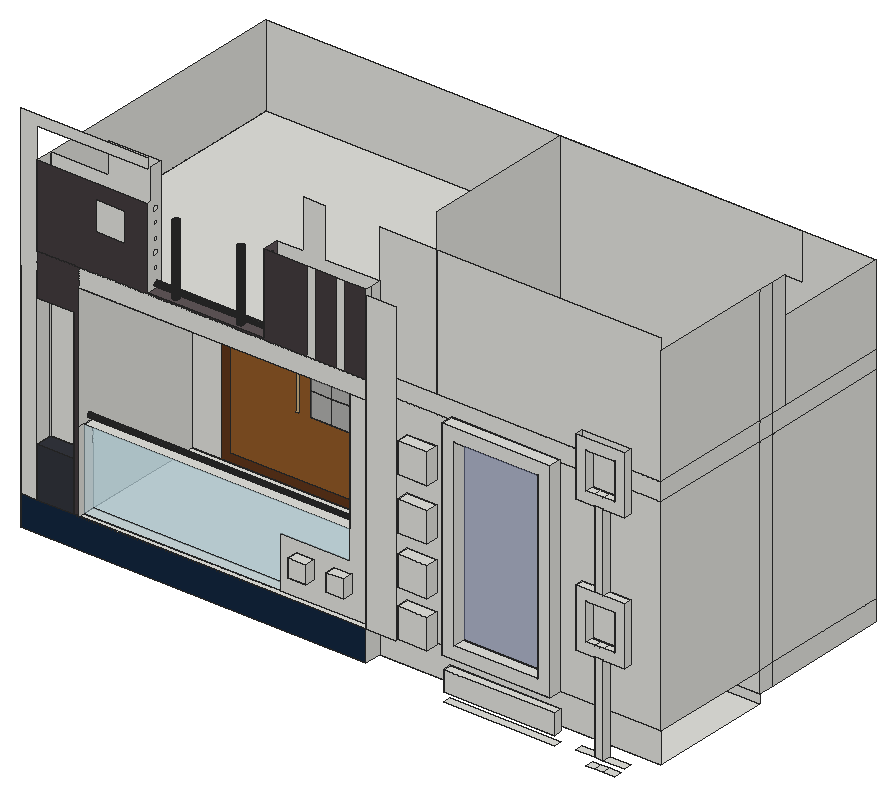
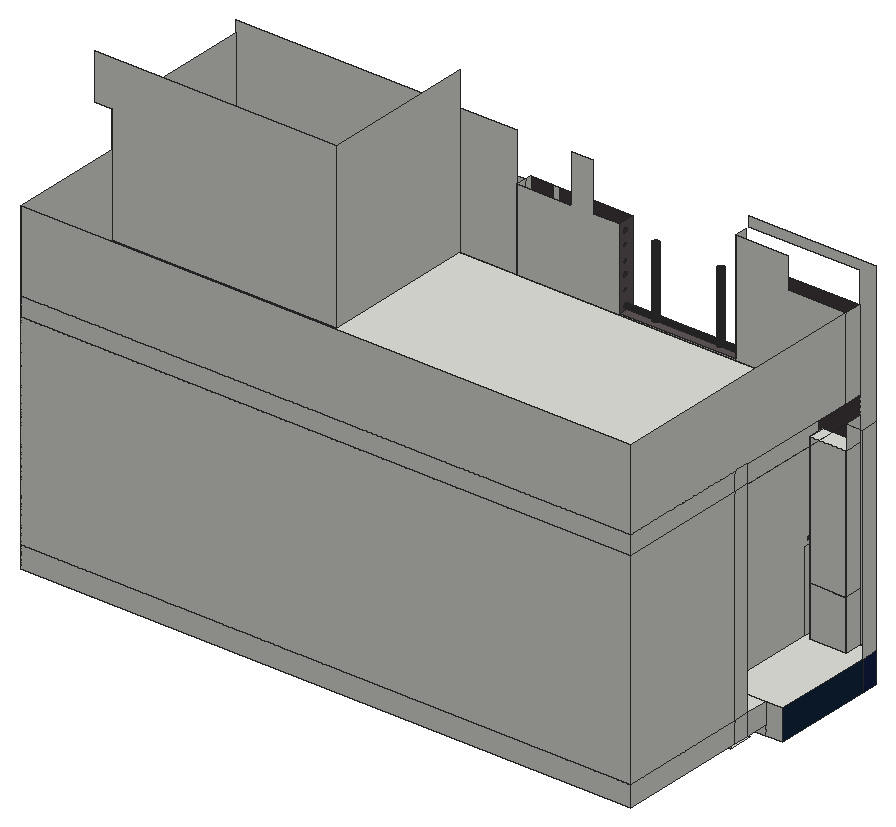
# SketchUp Ruby script. Lengths in inches.
U = 1.inch
M = Sketchup.active_model
def pt(a) = Geom::Point3d.new(a.map { |v| v * U })
def face(e, loops, mat)
  f = e.add_face(loops[0].map { |a| pt(a) })
  loops[1..].each { |l| e.add_face(l.map { |a| pt(a) }).erase! }
  f.material = f.back_material = mat if mat
  f
end
# faces: each face lists its corners as indices into pts; further lists are holes
def faces(e, pts, list, mat = nil) = list.each { |f| face(e, (f[0].is_a?(Array) ? f : [f]).map { |l| l.map { |i| pts[i] } }, mat) }
# xy, xz, yz: faces in a plane at the given z, y or x. An outline is a flat list of corners, or four numbers for a rectangle; further outlines are holes
def ring(l) = l.size == 4 ? [[l[0], l[1]], [l[2], l[1]], [l[2], l[3]], [l[0], l[3]]] : l.each_slice(2).to_a
def flat(e, list, mat, &to3) = list.each { |f| face(e, (f[0].is_a?(Array) ? f : [f]).map { |l| ring(l).map { |u, v| to3.(u, v) } }, mat) }
def xy(e, z, list, mat = nil) = flat(e, list, mat) { |x, y| [x, y, z] }
def xz(e, y, list, mat = nil) = flat(e, list, mat) { |x, z| [x, y, z] }
def yz(e, x, list, mat = nil) = flat(e, list, mat) { |y, z| [x, y, z] }
def lines(e, pts, list) = list.each { |a, b| e.add_line(pt(pts[a]), pt(pts[b])) }
# prism: a flat outline (further loops are holes) pulled along v
def prism(e, loops, v, mat = nil)
  f = face(e, loops, mat); d = Geom::Vector3d.new(v.map { |x| x * U })
  f.pushpull(f.normal.samedirection?(d) ? d.length : -d.length)
end
def box(e, o, s, mat = nil) = prism(e, [[o, [o[0] + s[0], o[1], o[2]], [o[0] + s[0], o[1] + s[1], o[2]], [o[0], o[1] + s[1], o[2]]]], [0, 0, s[2]], mat)
def at(x, y, z, deg = 0) = Geom::Transformation.translation(pt([x, y, z])) * Geom::Transformation.rotation(ORIGIN, Z_AXIS, deg.degrees)
def axes(o, x, y, z) = Geom::Transformation.new([*x, 0, *y, 0, *z, 0, *pt(o).to_a, 1])
def part(name) = M.definitions.add(name)
# library, detail: a bought-in or finely detailed component or shape, given as its bounding box
def library(name, o, s) = part(name).tap { |d| box(d.entities, o, s) }
def detail(e, o, s) = box(e.add_group.entities, o, s)
def put(e, d, t, mat = nil) = e.add_instance(d, t).tap { |i| i.material = mat if mat }
def group(e, t, mat = nil) = e.add_group.tap { |g| g.transformation = t; g.material = mat if mat }.entities
root = M.entities
M.materials.add("[Asphalt New]").color = [96, 86, 89]
M.materials.add("[Asphalt New]1").color = [67, 60, 62]
M.materials.add("[Carrera Marble]").color = [19, 39, 63]
M.materials.add("[Color M07]").color = [58, 58, 58]
M.materials.add("[Formica Laminate Dark]").color = [50, 53, 60]
M.materials.add("[Granite Dark Gray]").color = [18, 32, 73]
M.materials.add("[Translucent Glass Gray]").color = [128, 128, 128]
M.materials["[Translucent Glass Gray]"].alpha = 0.5
M.materials.add("[Translucent Glass Safety]").color = [213, 245, 255]
M.materials["[Translucent Glass Safety]"].alpha = 0.5
M.materials.add("[Translucent Glass Sky Reflection]").color = [126, 138, 183]
M.materials["[Translucent Glass Sky Reflection]"].alpha = 0.52
M.materials.add("[Wood Cherry Original]").color = [96, 54, 26]
M.materials.add("[Wood Floor Light]").color = [204, 176, 127]
M.materials.add("[Wood Floor Parquet]").color = [145, 89, 39]
box(root,[294.43,147.85,88.67],[58.93,4.5,10.68])
box(root,[271.51,145.85,106.65],[15.82,6.5,15.81])
box(root,[271.51,145.85,131.4],[15.82,6.5,15.81])
box(root,[271.51,145.85,157.4],[15.82,6.5,15.81])
box(root,[271.51,145.85,185.28],[15.82,6.5,15.81])
xy(root,80.14,[[370.09,148.04,374.5,152.35],[374.5,148.04,379.09,152.35],[379.09,148.04,385.11,152.35]])
xy(root,81.17,[[83.43,214.25,224.39,226.93]])
xy(root,83.85,[[294.43,147.85,353.36,152.35]])
xy(root,84.875,[[65.99,152.35,65.99,214.25,241.35,214.25,241.35,226.93,399.27,226.93,399.27,161.35,249.72,161.35,249.72,152.35]])
xy(root,85.66,[[364.57,148.04,374.5,152.35],[374.5,148.04,379.09,152.35],[379.09,148.04,390.63,152.35]])
xy(root,89.9375,[[74.99,214.25,241.35,226.93],[74.99,226.93,399.27,234.75],[74.99,234.75,399.27,304.28]])
xy(root,101,[[65.99,152.35,74.71,152.35,74.71,161.47,94.21,161.47,94.21,152.35,97.3,152.35,97.3,214.25,65.99,214.25],[74.71,152.35,94.21,161.47],[97.3,152.35,249.72,155.29],[97.3,155.29,249.72,161.35],[97.3,161.35,399.27,226.93],
  [74.99,214.25,97.3,226.93],[74.99,226.93,399.27,234.75],[74.99,234.75,399.27,304.28]])
xy(root,107.34,[[295.03,145.79,352.78,152.35]])
xy(root,112.78,[[210.38,149.85,219.82,155.29],[230.45,149.85,239.88,155.29]])
xy(root,113.91,[[301.6,145.79,346.21,152.35]])
xy(root,122.22,[[210.38,149.85,219.82,155.29],[230.45,149.85,239.88,155.29]])
xy(root,127.5,[[74.71,152.35,94.21,161.47]],"[Formica Laminate Dark]")
xy(root,133.35,[[364.57,148.04,374.5,152.35],[374.5,148.04,379.09,152.35],[379.09,148.04,390.63,152.35]])
xy(root,138.86,[[370.09,148.04,374.5,152.35],[374.5,148.04,379.09,152.35],[379.09,148.04,385.11,152.35]])
xy(root,143.5625,[[97.3,155.29,238.69,161.35]])
xy(root,158.64,[[370.09,148.04,374.5,152.35],[374.5,148.04,379.09,152.35],[379.09,148.04,385.11,152.35]])
xy(root,164.16,[[364.57,148.04,374.5,152.35],[374.5,148.04,379.09,152.35],[379.09,148.04,390.63,152.35]])
xy(root,197.27,[[74.71,152.35,94.21,161.47]])
xy(root,205.28,[[364.57,148.04,374.5,152.35],[374.5,148.04,379.09,152.35],[379.09,148.04,390.63,152.35]])
xy(root,209.9375,[[97.3,152.35,97.3,226.93,399.27,226.93,399.27,161.35,238.69,161.35,238.69,152.35],[238.69,152.35,249.72,155.29],[238.69,155.29,249.72,161.35],[74.99,226.93,399.27,234.75],[74.99,234.75,399.27,304.28]])
xy(root,210.8,[[370.09,148.04,374.5,152.35],[374.5,148.04,379.09,152.35],[379.09,148.04,385.11,152.35]])
xy(root,211.08,[[301.6,145.79,346.21,152.35]])
xy(root,217.65,[[295.03,145.79,352.78,152.35]])
xy(root,219.625,[[74.99,152.35,249.72,161.35],[74.99,161.35,280.02,161.35,280.02,243.33,399.27,243.33,399.27,304.28,74.99,304.28],[280.02,161.35,399.27,243.33]])
xy(root,220.1875,[[145.55,154.65,145.15,154.7,144.77,154.86,144.45,155.11,144.2,155.43,144.04,155.81,143.99,156.21,144.04,156.62,144.2,156.99,144.45,157.32,144.77,157.57,145.15,157.72,145.55,157.77,145.96,157.72,146.33,157.57,146.66,157.32,146.9,156.99,147.0625,156.62,147.11,156.21,147.0625,155.81,146.9,155.43,146.66,155.11,146.33,154.86,145.96,154.7],[180.11,154.65,179.71,154.7,179.33,154.86,179.01,155.11,178.76,155.43,178.6,155.81,178.55,156.21,178.6,156.62,178.76,156.99,179.01,157.32,179.33,157.57,179.71,157.72,180.11,157.77,180.52,157.72,180.9,157.57,181.22,157.32,181.47,156.99,181.625,156.62,181.68,156.21,181.625,155.81,181.47,155.43,181.22,155.11,180.9,154.86,180.52,154.7]])
xy(root,220.1875,[[[133.58,152.35,195.29,161.35],[145.55,154.65,145.15,154.7,144.77,154.86,144.45,155.11,144.2,155.43,144.04,155.81,143.99,156.21,144.04,156.62,144.2,156.99,144.45,157.32,144.77,157.57,145.15,157.72,145.55,157.77,145.96,157.72,146.33,157.57,146.66,157.32,146.9,156.99,147.0625,156.62,147.11,156.21,147.0625,155.81,146.9,155.43,146.66,155.11,146.33,154.86,145.96,154.7],[180.11,154.65,179.71,154.7,179.33,154.86,179.01,155.11,178.76,155.43,178.6,155.81,178.55,156.21,178.6,156.62,178.76,156.99,179.01,157.32,179.33,157.57,179.71,157.72,180.11,157.77,180.52,157.72,180.9,157.57,181.22,157.32,181.47,156.99,181.625,156.62,181.68,156.21,181.625,155.81,181.47,155.43,181.22,155.11,180.9,154.86,180.52,154.7]]],"[Asphalt New]")
xz(root,145.79,[[[295.03,107.34,352.78,217.65],[301.6,113.91,346.21,211.08]]])
xz(root,148.04,[[374.5,85.66,379.09,133.35],[[364.57,133.35,390.63,164.16],[370.09,138.86,385.11,158.64]],[374.5,164.16,379.09,205.28],[[364.57,205.28,390.63,236.1],[370.09,210.8,385.11,230.58]]])
xz(root,149.85,[[210.38,112.78,219.82,122.22],[230.45,112.78,239.88,122.22]])
xz(root,152.35,[[374.5,85.66,379.09,133.35],[65.99,101,74.71,101,74.71,209.9375,74.99,219.625,74.99,279.1,133.58,279.1,133.58,284.4375,65.99,284.4375],[249.72,101,265.65,260.08],[[295.03,107.34,352.78,217.65],[301.6,113.91,346.21,211.08]],[[364.57,133.35,390.63,164.16],[370.09,138.86,385.11,158.64]],
  [370.09,138.86,385.11,158.64],[374.5,164.16,379.09,205.28],[[364.57,205.28,390.63,236.1],[370.09,210.8,385.11,230.58]],[97.3,209.9375,249.72,219.625],[370.09,210.8,385.11,230.58],
  [218.4,219.625,222.46,262.6875],[233.96,219.625,238.02,262.6875]])
xz(root,152.35,[[94.21,101,97.3,101,97.3,219.625,74.99,219.625,74.71,209.9375,74.71,197.27,94.21,197.27],[[74.99,219.625,218.4,219.625,218.4,262.6875,195.29,262.6875,195.29,220.1875,133.58,220.1875,133.58,262.6875,74.99,262.6875],[105.86,239.3,121.54,254.99]],[222.46,219.625,233.96,262.6875],[238.02,219.625,249.72,262.6875]],"[Asphalt New]1")
xz(root,152.35,[[65.99,84.875,249.72,101]],"[Carrera Marble]")
xz(root,152.35,[[74.71,101,94.21,127.5]],"[Formica Laminate Dark]")
xz(root,152.35,[[301.6,113.91,346.21,211.08]],"[Translucent Glass Sky Reflection]")
xz(root,155.29,[[[201.94,101,249.72,101,249.72,209.9375,238.69,209.9375,238.69,128.1875,201.94,128.1875],[210.38,112.78,219.82,122.22],[230.45,112.78,239.88,122.22]],[210.38,112.78,219.82,122.22],[230.45,112.78,239.88,122.22]])
xz(root,155.29,[[97.3,101,201.94,101,201.94,128.1875,238.69,128.1875,238.69,143.5625,97.3,143.5625]],"[Translucent Glass Safety]")
xz(root,161.35,[[249.72,84.875,399.27,101],[249.72,101,399.27,209.9375],[249.72,209.9375,399.27,219.625],[74.99,219.625,74.99,262.6875,106.04,262.6875,106.04,279.1,133.58,279.1,133.58,220.1875,195.29,220.1875,195.29,262.6875,209.34,262.6875,209.34,288.3125,220.78,288.3125,220.78,262.6875,249.72,262.6875,249.72,219.625],[249.72,219.625,280.02,288.3125],
  [280.02,219.625,399.27,288.3125]])
xz(root,161.35,[[97.3,101,97.3,143.5625,238.69,143.5625,238.69,209.9375,249.72,209.9375,249.72,101]],"[Translucent Glass Safety]")
xz(root,161.47,[[74.71,101,94.21,127.5],[74.71,127.5,94.21,197.27]])
xz(root,214.25,[[65.99,84.875,74.99,101],[74.99,84.875,241.35,89.9375]])
xz(root,226.93,[[83.43,81.17,224.39,89.9375],[241.35,84.875,399.27,89.9375],[74.99,89.9375,399.27,101],[74.99,101,97.3,209.9375],[97.3,101,113.07,101,113.07,192.125,188.51,192.125,188.51,101,399.27,101,399.27,209.9375,97.3,209.9375]])
xz(root,226.93,[[160.69,137.52,172.08,150.1],[172.08,137.52,183.47,150.1],[160.69,150.1,172.08,162.67],[172.08,150.1,183.47,162.67],[160.69,162.67,172.08,175.46],
  [172.08,162.67,183.47,175.46],[160.69,175.46,172.08,187.08],[172.08,175.46,183.47,187.08]],"[Translucent Glass Gray]")
xz(root,226.93,[[[113.07,101,188.51,192.125],[118.11,106.04,183.47,187.08]]],"[Wood Cherry Original]")
xz(root,226.93,[[152.7,137.52,155.05,157.98]],"[Wood Floor Light]")
xz(root,226.93,[[[118.11,106.04,183.47,106.04,183.47,137.52,160.69,137.52,160.69,187.08,118.11,187.08],[152.7,137.52,155.05,157.98]]],"[Wood Floor Parquet]")
xz(root,234.75,[[74.99,89.9375,399.27,101],[74.99,101,399.27,209.9375]])
xz(root,243.33,[[280.02,219.625,280.02,306.375,408.27,306.375,408.27,281.9375,399.27,281.9375,399.27,219.625]])
xz(root,304.28,[[74.99,89.9375,399.27,101],[74.99,101,399.27,209.9375],[74.99,209.9375,399.27,219.625],[74.99,219.625,399.27,262.6875]])
yz(root,65.99,[[152.35,101,161.35,209.9375]])
yz(root,65.99,[[161.35,84.875,214.25,101]],"[Carrera Marble]")
yz(root,65.99,[[152.35,84.875,161.35,101]],"[Granite Dark Gray]")
yz(root,74.71,[[152.35,101,161.35,127.5],[161.35,101,161.47,127.5],[152.35,127.5,161.35,197.27],[161.35,127.5,161.47,197.27],[152.35,197.27,161.35,209.9375]])
yz(root,74.99,[[214.25,89.9375,226.93,101],[226.93,89.9375,234.75,101],[234.75,89.9375,304.28,101],[226.93,101,234.75,209.9375],[234.75,101,304.28,209.9375],
  [226.93,209.9375,234.75,219.625],[234.75,209.9375,304.28,219.625],[152.35,219.625,161.35,262.6875],[161.35,219.625,304.28,262.6875]])
yz(root,94.21,[[152.35,101,161.47,127.5],[152.35,127.5,161.47,197.27]])
yz(root,97.3,[[152.35,101,155.29,143.5625],[[161.35,101,226.93,101,226.93,209.9375,152.35,209.9375,152.35,143.5625,161.35,143.5625],[158.43,145.79,158.16,145.83,157.9,145.9375,157.68,146.11,157.51,146.33,157.41,146.58,157.37,146.86,157.41,147.13,157.51,147.39,157.68,147.61,157.9,147.78,158.16,147.88,158.43,147.92,158.71,147.88,158.96,147.78,159.18,147.61,159.35,147.39,159.46,147.13,159.49,146.86,159.46,146.58,159.35,146.33,159.18,146.11,158.96,145.9375,158.71,145.83]],[155.29,101,161.35,143.5625]])
yz(root,133.58,[[[152.35,220.1875,161.35,220.1875,161.35,279.1,154.79,279.1,154.79,262.6875,152.35,262.6875],[157.4,256.53,156.97,256.58,156.5625,256.75,156.21,257.02,155.94,257.37,155.77,257.78,155.72,258.21,155.77,258.65,155.94,259.06,156.21,259.41,156.5625,259.68,156.97,259.84,157.4,259.9,157.84,259.84,158.25,259.68,158.6,259.41,158.87,259.06,159.03,258.65,159.09,258.21,159.03,257.78,158.87,257.37,158.6,257.02,158.25,256.75,157.84,256.58],[157.4,235.59,156.97,235.65,156.5625,235.82,156.21,236.08,155.94,236.43,155.77,236.84,155.72,237.28,155.77,237.71,155.94,238.12,156.21,238.47,156.5625,238.74,156.97,238.91,157.4,238.96,157.84,238.91,158.25,238.74,158.6,238.47,158.87,238.12,159.03,237.71,159.09,237.28,159.03,236.84,158.87,236.43,158.6,236.08,158.25,235.82,157.84,235.65],[157.64,221.32,157.33,221.36,157.04,221.47,156.8,221.66,156.61,221.91,156.49,222.2,156.45,222.5,156.49,222.8125,156.61,223.1,156.8,223.34,157.04,223.53,157.33,223.65,157.64,223.69,157.94,223.65,158.23,223.53,158.48,223.34,158.67,223.1,158.78,222.8125,158.82,222.5,158.78,222.2,158.67,221.91,158.48,221.66,158.23,221.47,157.94,221.36],[157.64,228.69,157.33,228.73,157.04,228.85,156.8,229.04,156.61,229.28,156.49,229.57,156.45,229.88,156.49,230.1875,156.61,230.47,156.8,230.72,157.04,230.91,157.33,231.03,157.64,231.07,157.94,231.03,158.23,230.91,158.48,230.72,158.67,230.47,158.78,230.1875,158.82,229.88,158.78,229.57,158.67,229.28,158.48,229.04,158.23,228.85,157.94,228.73],[157.64,242.44,157.33,242.48,157.04,242.6,156.8,242.79,156.61,243.03,156.49,243.32,156.45,243.63,156.49,243.9375,156.61,244.22,156.8,244.47,157.04,244.66,157.33,244.78,157.64,244.82,157.94,244.78,158.23,244.66,158.48,244.47,158.67,244.22,158.78,243.9375,158.82,243.63,158.78,243.32,158.67,243.03,158.48,242.79,158.23,242.6,157.94,242.48],[157.64,250.38,157.33,250.42,157.04,250.54,156.8,250.73,156.61,250.97,156.49,251.26,156.45,251.57,156.49,251.875,156.61,252.16,156.8,252.41,157.04,252.59,157.33,252.71,157.64,252.75,157.94,252.71,158.23,252.59,158.48,252.41,158.67,252.16,158.78,251.875,158.82,251.57,158.78,251.26,158.67,250.97,158.48,250.73,158.23,250.54,157.94,250.42]]])
yz(root,195.29,[[[152.35,220.1875,161.35,262.6875],[157.4,235.59,157.84,235.65,158.25,235.82,158.6,236.08,158.87,236.43,159.03,236.84,159.09,237.28,159.03,237.71,158.87,238.12,158.6,238.47,158.25,238.74,157.84,238.91,157.4,238.96,156.97,238.91,156.5625,238.74,156.21,238.47,155.94,238.12,155.77,237.71,155.72,237.28,155.77,236.84,155.94,236.43,156.21,236.08,156.5625,235.82,156.97,235.65],[157.4,256.53,157.84,256.58,158.25,256.75,158.6,257.02,158.87,257.37,159.03,257.78,159.09,258.21,159.03,258.65,158.87,259.06,158.6,259.41,158.25,259.68,157.84,259.84,157.4,259.9,156.97,259.84,156.5625,259.68,156.21,259.41,155.94,259.06,155.77,258.65,155.72,258.21,155.77,257.78,155.94,257.37,156.21,257.02,156.5625,256.75,156.97,256.58],[157.64,242.44,157.94,242.48,158.23,242.6,158.48,242.79,158.67,243.03,158.78,243.32,158.82,243.63,158.78,243.9375,158.67,244.22,158.48,244.47,158.23,244.66,157.94,244.78,157.64,244.82,157.33,244.78,157.04,244.66,156.8,244.47,156.61,244.22,156.49,243.9375,156.45,243.63,156.49,243.32,156.61,243.03,156.8,242.79,157.04,242.6,157.33,242.48],[157.64,250.38,157.94,250.42,158.23,250.54,158.48,250.73,158.67,250.97,158.78,251.26,158.82,251.57,158.78,251.875,158.67,252.16,158.48,252.41,158.23,252.59,157.94,252.71,157.64,252.75,157.33,252.71,157.04,252.59,156.8,252.41,156.61,252.16,156.49,251.875,156.45,251.57,156.49,251.26,156.61,250.97,156.8,250.73,157.04,250.54,157.33,250.42],[157.64,228.69,157.94,228.73,158.23,228.85,158.48,229.04,158.67,229.28,158.78,229.57,158.82,229.88,158.78,230.1875,158.67,230.47,158.48,230.72,158.23,230.91,157.94,231.03,157.64,231.07,157.33,231.03,157.04,230.91,156.8,230.72,156.61,230.47,156.49,230.1875,156.45,229.88,156.49,229.57,156.61,229.28,156.8,229.04,157.04,228.85,157.33,228.73],[157.64,221.32,157.94,221.36,158.23,221.47,158.48,221.66,158.67,221.91,158.78,222.2,158.82,222.5,158.78,222.8125,158.67,223.1,158.48,223.34,158.23,223.53,157.94,223.65,157.64,223.69,157.33,223.65,157.04,223.53,156.8,223.34,156.61,223.1,156.49,222.8125,156.45,222.5,156.49,222.2,156.61,221.91,156.8,221.66,157.04,221.47,157.33,221.36]],[157.64,221.32,157.94,221.36,158.23,221.47,158.48,221.66,158.67,221.91,158.78,222.2,158.82,222.5,158.78,222.8125,158.67,223.1,158.48,223.34,158.23,223.53,157.94,223.65,157.64,223.69,157.33,223.65,157.04,223.53,156.8,223.34,156.61,223.1,156.49,222.8125,156.45,222.5,156.49,222.2,156.61,221.91,156.8,221.66,157.04,221.47,157.33,221.36]],"[Asphalt New]")
yz(root,210.38,[[149.85,112.78,155.29,122.22]])
yz(root,219.82,[[149.85,112.78,155.29,122.22]])
yz(root,230.45,[[149.85,112.78,155.29,122.22]])
yz(root,238.69,[[[155.29,143.5625,161.35,209.9375],[158.43,145.79,158.71,145.83,158.96,145.9375,159.18,146.11,159.35,146.33,159.46,146.58,159.49,146.86,159.46,147.13,159.35,147.39,159.18,147.61,158.96,147.78,158.71,147.88,158.43,147.92,158.16,147.88,157.9,147.78,157.68,147.61,157.51,147.39,157.41,147.13,157.37,146.86,157.41,146.58,157.51,146.33,157.68,146.11,157.9,145.9375,158.16,145.83]],[158.43,145.79,158.71,145.83,158.96,145.9375,159.18,146.11,159.35,146.33,159.46,146.58,159.49,146.86,159.46,147.13,159.35,147.39,159.18,147.61,158.96,147.78,158.71,147.88,158.43,147.92,158.16,147.88,157.9,147.78,157.68,147.61,157.51,147.39,157.41,147.13,157.37,146.86,157.41,146.58,157.51,146.33,157.68,146.11,157.9,145.9375,158.16,145.83]])
yz(root,239.88,[[149.85,112.78,155.29,122.22]])
yz(root,241.35,[[214.25,84.875,226.93,89.9375]])
yz(root,249.72,[[152.35,84.875,161.35,101],[152.35,101,155.29,209.9375],[155.29,101,161.35,209.9375],[152.35,209.9375,155.29,219.625],[155.29,209.9375,161.35,219.625],
  [152.35,219.625,155.29,262.6875],[155.29,219.625,161.35,262.6875]])
yz(root,280.02,[[161.35,219.625,243.33,306.375]])
yz(root,295.03,[[145.79,107.34,152.35,217.65]])
yz(root,301.6,[[145.79,113.91,152.35,211.08]])
yz(root,346.21,[[145.79,113.91,152.35,211.08]])
yz(root,352.78,[[145.79,107.34,152.35,217.65]])
yz(root,364.57,[[148.04,133.35,152.35,164.16],[148.04,205.28,152.35,236.1]])
yz(root,370.09,[[148.04,138.86,152.35,158.64],[148.04,210.8,152.35,230.58]])
yz(root,374.5,[[148.04,85.66,152.35,133.35],[148.04,164.16,152.35,205.28]])
yz(root,379.09,[[148.04,85.66,152.35,133.35],[148.04,164.16,152.35,205.28]])
yz(root,385.11,[[148.04,138.86,152.35,158.64],[148.04,210.8,152.35,230.58]])
yz(root,390.63,[[148.04,133.35,152.35,164.16],[148.04,205.28,152.35,236.1]])
yz(root,399.27,[[226.93,89.9375,234.75,101],[234.75,89.9375,304.28,101],[161.35,101,226.93,209.9375],[226.93,101,234.75,209.9375],[234.75,101,304.28,209.9375],
  [161.35,209.9375,226.93,219.625],[226.93,209.9375,234.75,219.625],[234.75,209.9375,304.28,219.625],[161.35,219.625,226.93,281.9375],[226.93,219.625,234.75,281.9375],
  [234.75,219.625,243.33,281.9375],[243.33,219.625,304.28,262.6875]])
p = [[238.69,158.16,145.83],[238.69,157.9,145.9375],[97.3,157.9,145.9375],[97.3,158.16,145.83],[238.69,158.43,145.79],[97.3,158.43,145.79],
  [238.69,158.71,145.83],[97.3,158.71,145.83],[238.69,158.96,145.9375],[97.3,158.96,145.9375],[238.69,157.68,146.11],[97.3,157.68,146.11],
  [238.69,159.18,146.11],[97.3,159.18,146.11],[238.69,157.51,146.33],[97.3,157.51,146.33],[238.69,159.35,146.33],[97.3,159.35,146.33],
  [238.69,157.41,146.58],[97.3,157.41,146.58],[238.69,159.46,146.58],[97.3,159.46,146.58],[238.69,157.37,146.86],[97.3,157.37,146.86],
  [238.69,159.49,146.86],[97.3,159.49,146.86],[238.69,157.41,147.13],[97.3,157.41,147.13],[238.69,159.46,147.13],[97.3,159.46,147.13],
  [238.69,157.51,147.39],[97.3,157.51,147.39],[238.69,159.35,147.39],[97.3,159.35,147.39],[238.69,157.68,147.61],[97.3,157.68,147.61],
  [238.69,159.18,147.61],[97.3,159.18,147.61],[238.69,157.9,147.78],[97.3,157.9,147.78],[238.69,158.96,147.78],[97.3,158.96,147.78],
  [238.69,158.16,147.88],[97.3,158.16,147.88],[238.69,158.71,147.88],[97.3,158.71,147.88],[238.69,158.43,147.92],[97.3,158.43,147.92],
  [145.15,154.7,220.1875],[145.55,154.65,220.1875],[145.55,154.65,257.37],[145.15,154.7,257.37],[145.96,154.7,220.1875],[145.96,154.7,257.37],
  [179.71,154.7,220.1875],[180.11,154.65,220.1875],[180.11,154.65,257.37],[179.71,154.7,257.37],[180.52,154.7,220.1875],[180.52,154.7,257.37],
  [144.77,154.86,220.1875],[144.77,154.86,257.37],[146.33,154.86,220.1875],[146.33,154.86,257.37],[179.33,154.86,220.1875],[179.33,154.86,257.37],
  [180.9,154.86,220.1875],[180.9,154.86,257.37],[144.45,155.11,220.1875],[144.45,155.11,257.37],[146.66,155.11,220.1875],[146.66,155.11,257.37],
  [179.01,155.11,220.1875],[179.01,155.11,257.37],[181.22,155.11,220.1875],[181.22,155.11,257.37],[144.2,155.43,220.1875],[144.2,155.43,257.37],
  [146.9,155.43,220.1875],[146.9,155.43,257.37],[178.76,155.43,220.1875],[178.76,155.43,257.37],[181.47,155.43,220.1875],[181.47,155.43,257.37],
  [144.04,155.81,220.1875],[144.04,155.81,257.37],[147.0625,155.81,220.1875],[147.0625,155.81,257.37],[178.6,155.81,220.1875],[178.6,155.81,257.37],
  [181.625,155.81,220.1875],[181.625,155.81,257.37],[143.99,156.21,220.1875],[144.02,155.94,257.37],[143.99,156.21,257.37],[143.99,156.21,257.02],
  [143.99,156.21,238.47],[143.99,156.21,236.08],[147.11,156.21,220.1875],[147.11,156.21,236.08],[147.11,156.21,238.47],[147.11,156.21,257.02],
  [147.11,156.21,257.37],[147.08,155.94,257.37],[178.55,156.21,220.1875],[178.59,155.94,257.37],[178.55,156.21,257.37],[178.55,156.21,257.02],
  [178.55,156.21,238.47],[178.55,156.21,236.08],[181.68,156.21,220.1875],[181.68,156.21,236.08],[181.68,156.21,238.47],[181.68,156.21,257.02],
  [181.68,156.21,257.37],[181.64,155.94,257.37],[144.04,156.62,220.1875],[144.04,156.62,257.37],[147.0625,156.62,220.1875],[147.0625,156.62,257.37],
  [178.6,156.62,220.1875],[178.6,156.62,257.37],[181.625,156.62,220.1875],[181.625,156.62,257.37],[144.2,156.99,220.1875],[144.2,156.99,257.37],
  [146.9,156.99,220.1875],[146.9,156.99,257.37],[178.76,156.99,220.1875],[178.76,156.99,257.37],[181.47,156.99,220.1875],[181.47,156.99,257.37],
  [144.45,157.32,220.1875],[144.45,157.32,257.37],[146.66,157.32,220.1875],[146.66,157.32,257.37],[179.01,157.32,220.1875],[179.01,157.32,257.37],
  [181.22,157.32,220.1875],[181.22,157.32,257.37],[144.77,157.57,220.1875],[144.77,157.57,257.37],[146.33,157.57,220.1875],[146.33,157.57,257.37],
  [179.33,157.57,220.1875],[179.33,157.57,257.37],[180.9,157.57,220.1875],[180.9,157.57,257.37],[145.15,157.72,220.1875],[145.15,157.72,257.37],
  [145.96,157.72,220.1875],[145.96,157.72,257.37],[179.71,157.72,220.1875],[179.71,157.72,257.37],[180.52,157.72,220.1875],[180.52,157.72,257.37],
  [145.55,157.77,220.1875],[145.55,157.77,257.37],[180.11,157.77,220.1875],[180.11,157.77,257.37],[195.29,157.64,221.32],[195.29,157.33,221.36],
  [133.58,157.33,221.36],[133.58,157.64,221.32],[195.29,157.94,221.36],[133.58,157.94,221.36],[195.29,157.04,221.47],[133.58,157.04,221.47],
  [195.29,158.23,221.47],[133.58,158.23,221.47],[195.29,156.8,221.66],[133.58,156.8,221.66],[195.29,158.48,221.66],[133.58,158.48,221.66],
  [195.29,156.61,221.91],[133.58,156.61,221.91],[195.29,158.67,221.91],[133.58,158.67,221.91],[195.29,156.49,222.2],[133.58,156.49,222.2],
  [195.29,158.78,222.2],[133.58,158.78,222.2],[195.29,156.45,222.5],[133.58,156.45,222.5],[195.29,158.82,222.5],[133.58,158.82,222.5],
  [195.29,156.49,222.8125],[133.58,156.49,222.8125],[195.29,158.78,222.8125],[133.58,158.78,222.8125],[195.29,156.61,223.1],[133.58,156.61,223.1],
  [195.29,158.67,223.1],[133.58,158.67,223.1],[195.29,156.8,223.34],[133.58,156.8,223.34],[195.29,158.48,223.34],[133.58,158.48,223.34],
  [195.29,157.04,223.53],[133.58,157.04,223.53],[195.29,158.23,223.53],[133.58,158.23,223.53],[195.29,157.33,223.65],[133.58,157.33,223.65],
  [195.29,157.94,223.65],[133.58,157.94,223.65],[195.29,157.64,223.69],[133.58,157.64,223.69],[65.99,161.35,209.9375],[74.71,161.35,209.9375],
  [74.71,161.35,89.9375],[74.71,161.35,101],[74.99,226.93,209.9375],[74.99,152.35,209.9375],[74.71,152.35,209.9375]]
faces(root,p,[[0,1,2,3],[4,0,3,5],[6,4,5,7],[8,6,7,9],[1,10,11,2],[12,8,9,13],[10,14,15,11],[16,12,13,17],
  [14,18,19,15],[20,16,17,21],[18,22,23,19],[24,20,21,25],[22,26,27,23],[28,24,25,29],[26,30,31,27],[32,28,29,33],
  [30,34,35,31],[36,32,33,37],[34,38,39,35],[40,36,37,41],[38,42,43,39],[44,40,41,45],[42,46,47,43],[46,44,45,47]],"[Formica Laminate Dark]")
faces(root,p,[[48,49,50,51],[49,52,53,50],[54,55,56,57],[55,58,59,56],[60,48,51,61],[52,62,63,53],[64,54,57,65],[58,66,67,59],
  [68,60,61,69],[62,70,71,63],[72,64,65,73],[66,74,75,67],[76,68,69,77],[70,78,79,71],[80,72,73,81],[74,82,83,75],
  [84,76,77,85],[78,86,87,79],[88,80,81,89],[82,90,91,83],[92,84,85,93,94,95,96,97],[86,98,99,100,101,102,103,87],[104,88,89,105,106,107,108,109],[90,110,111,112,113,114,115,91],
  [116,92,97,96,95,94,117],[98,118,119,102,101,100,99],[120,104,109,108,107,106,121],[110,122,123,114,113,112,111],[124,116,117,125],[118,126,127,119],[128,120,121,129],[122,130,131,123],
  [132,124,125,133],[126,134,135,127],[136,128,129,137],[130,138,139,131],[140,132,133,141],[134,142,143,135],[144,136,137,145],[138,146,147,139],
  [148,140,141,149],[142,150,151,143],[152,144,145,153],[146,154,155,147],[156,148,149,157],[150,156,157,151],[158,152,153,159],[154,158,159,155],
  [160,161,162,163],[164,160,163,165],[161,166,167,162],[168,164,165,169],[166,170,171,167],[172,168,169,173],[170,174,175,171],[176,172,173,177],
  [174,178,179,175],[180,176,177,181],[178,182,183,179],[184,180,181,185],[182,186,187,183],[188,184,185,189],[186,190,191,187],[192,188,189,193],
  [190,194,195,191],[196,192,193,197],[194,198,199,195],[200,196,197,201],[198,202,203,199],[204,200,201,205],[202,206,207,203],[206,204,205,207]],"[Color M07]")
lines(root,p,[[208,209],[210,211],[212,213],[214,213]])
